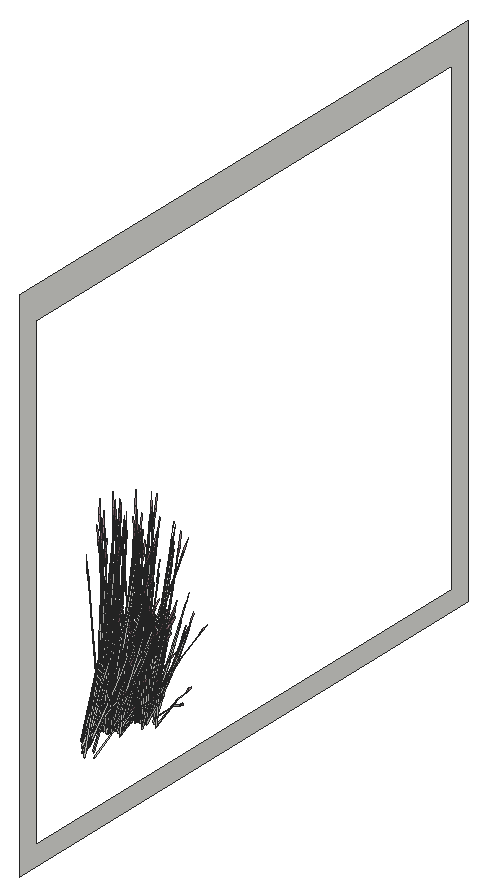
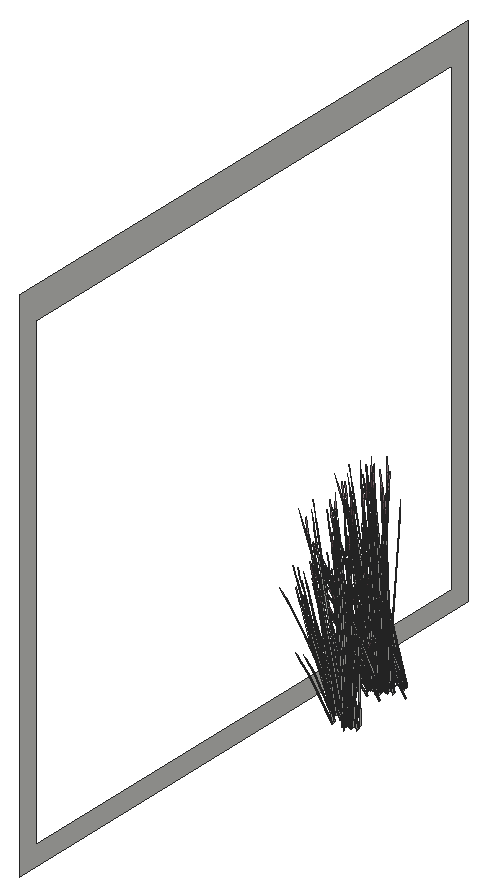
# SketchUp Ruby script. Lengths in inches.
U = 1.inch
M = Sketchup.active_model
def pt(a) = Geom::Point3d.new(a.map { |v| v * U })
def face(e, loops, mat)
  f = e.add_face(loops[0].map { |a| pt(a) })
  loops[1..].each { |l| e.add_face(l.map { |a| pt(a) }).erase! }
  f.material = f.back_material = mat if mat
  f
end
# faces: each face lists its corners as indices into pts; further lists are holes
def faces(e, pts, list, mat = nil) = list.each { |f| face(e, (f[0].is_a?(Array) ? f : [f]).map { |l| l.map { |i| pts[i] } }, mat) }
# xy, xz, yz: faces in a plane at the given z, y or x. An outline is a flat list of corners, or four numbers for a rectangle; further outlines are holes
def ring(l) = l.size == 4 ? [[l[0], l[1]], [l[2], l[1]], [l[2], l[3]], [l[0], l[3]]] : l.each_slice(2).to_a
def flat(e, list, mat, &to3) = list.each { |f| face(e, (f[0].is_a?(Array) ? f : [f]).map { |l| ring(l).map { |u, v| to3.(u, v) } }, mat) }
def xy(e, z, list, mat = nil) = flat(e, list, mat) { |x, y| [x, y, z] }
def xz(e, y, list, mat = nil) = flat(e, list, mat) { |x, z| [x, y, z] }
def yz(e, x, list, mat = nil) = flat(e, list, mat) { |y, z| [x, y, z] }
def lines(e, pts, list) = list.each { |a, b| e.add_line(pt(pts[a]), pt(pts[b])) }
# prism: a flat outline (further loops are holes) pulled along v
def prism(e, loops, v, mat = nil)
  f = face(e, loops, mat); d = Geom::Vector3d.new(v.map { |x| x * U })
  f.pushpull(f.normal.samedirection?(d) ? d.length : -d.length)
end
def box(e, o, s, mat = nil) = prism(e, [[o, [o[0] + s[0], o[1], o[2]], [o[0] + s[0], o[1] + s[1], o[2]], [o[0], o[1] + s[1], o[2]]]], [0, 0, s[2]], mat)
def at(x, y, z, deg = 0) = Geom::Transformation.translation(pt([x, y, z])) * Geom::Transformation.rotation(ORIGIN, Z_AXIS, deg.degrees)
def axes(o, x, y, z) = Geom::Transformation.new([*x, 0, *y, 0, *z, 0, *pt(o).to_a, 1])
def part(name) = M.definitions.add(name)
# library, detail: a bought-in or finely detailed component or shape, given as its bounding box
def library(name, o, s) = part(name).tap { |d| box(d.entities, o, s) }
def detail(e, o, s) = box(e.add_group.entities, o, s)
def put(e, d, t, mat = nil) = e.add_instance(d, t).tap { |i| i.material = mat if mat }
def group(e, t, mat = nil) = e.add_group.tap { |g| g.transformation = t; g.material = mat if mat }.entities
root = M.entities
M.materials.add("LightPink_Translucent").color = [144, 107, 117]
M.materials["LightPink_Translucent"].alpha = 0.75
c1 = part("blade")
p = [[2.15,0.21,22],[0,0.17,0],[0.09,0.45,0],[2.18,0.31,22],[2.29,0.31,22],[0.38,0.45,0],
  [2.48,0.24,33],[2.49,0.24,33],[2.48,0.22,33]]
faces(c1.entities,p,[[0,1,2,3],[4,5,2,3],[6,3,4,7],[8,0,3,6]])
c2 = part("seeds")
p = [[0.3,-0.1,1.38],[-0.01,-0.03,1.59],[-0.01,-0.03,0.03],[0.14,-0.07,-0.07],[0.29,-0.03,3],[0.15,0.01,3.11]]
faces(c2.entities,p,[[0,1,2,3],[1,0,4,5]],"LightPink_Translucent")
c3 = part("blade with seeds")
put(c3.entities,c1,at(0,0,0))
put(c3.entities,c2,axes([2.4,0.25,30.99],[1.5799,-0.05474,1.17369],[-0.12525,1.92788,0.29478],[-0.07173,-0.02425,1.56792]))
yz(root,366,[[[45,0,219,162],[51,6,213,151.99]]])
put(root,c3,axes([347.85,102.97,10.68],[-0.22982,-0.59576,-0.51099],[0.87033,-0.10422,-0.3958],[0.24941,-0.16002,0.97773]))
put(root,c3,axes([344.8,97.15,7],[0.00265,-0.07899,1.77383],[0.76665,-0.34851,-0.16761],[0.2663,0.12439,0.31391]))
put(root,c3,axes([347.41,96.85,3.79],[0.06518,-0.0942,1.76342],[0.82057,-0.27742,-0.26939],[0.24877,0.14358,0.30037]))
put(root,c3,axes([346.33,94.71,4.39],[0.32803,0.59738,-0.69212],[-0.94492,0.21515,-0.18165],[0.03626,0.20229,1.52773]))
put(root,c3,axes([346.13,96.41,6.97],[0.88277,-0.1551,-0.51099],[0.15442,0.58737,-0.3958],[0.23711,0.16832,0.97773]))
put(root,c3,axes([343.68,96.5,7.34],[0.2697,-0.50175,0.35414],[0.78684,0.14635,-0.4572],[0.07215,0.20201,0.87481]))
put(root,c3,axes([347.35,97,4.96],[-0.57368,-0.02046,1.0506],[0.37886,-0.43461,0.58006],[0.22663,0.15441,0.8241]))
put(root,c3,axes([345.7,96.89,7.02],[-0.4066,0.41448,0.0643],[-0.57901,-0.24131,0.50621],[0.18719,0.13288,0.77189]))
put(root,c3,axes([343.58,101.61,8.02],[0.83726,-0.32623,-0.49651],[0.50045,0.58498,0],[0.19069,-0.0743,1.57504]))
put(root,c3,axes([344.74,98.29,7.9375],[0.61821,-0.37431,-0.06488],[0.56645,0.40995,-0.29416],[0.03988,0.11616,0.97024]))
put(root,c3,axes([348.55,102.74,8.59],[-0.31959,-0.01933,1.43002],[-0.32741,-0.51843,-0.30754],[0.39262,-0.14666,0.61141]))
put(root,c3,axes([345.87,96.77,7.03],[-0.88979,0.14973,0.48003],[-0.15442,-0.58737,0.3958],[0.20926,0.17311,0.9933]))
put(root,c3,axes([344.57,102.95,8.06],[0.60257,-0.49041,-0.62353],[0.74854,0.44469,-0.16365],[0.24146,-0.12234,1.37633]))
put(root,c3,axes([348.92,101.79,8.77],[-0.29798,0.33213,1.1486],[-0.25612,-0.44624,0.84392],[0.24611,-0.11182,0.25299]))
put(root,c3,axes([345.48,95.95,4.88],[0.01579,-0.21629,1.43002],[0.75442,-0.24159,-0.30754],[0.23289,0.25887,0.61141]))
put(root,c3,axes([348.49,103.04,10.53],[0.77872,-0.09325,-0.35414],[0.20563,0.53305,0.4572],[0.22316,-0.14318,0.87481]))
put(root,c3,axes([343.42,96.71,7.33],[0.87543,-0.30377,-0.1216],[0.4302,0.53915,-0.67495],[0.1155,0.2272,1.02557]))
put(root,c3,axes([343.53,103.8125,8.21],[0.43405,-0.58792,-0.44739],[0.90188,0.28295,0.21531],[0,-0.13553,1.43643]))
put(root,c3,axes([343.92,103.52,8.67],[-0.10425,-0.7445,-0.29095],[1.08575,-0.04502,-0.50002],[0.19119,-0.09917,1.59708]))
put(root,c3,axes([343.58,96.83,3.79],[0.14478,-0.0355,1.76342],[0.8709,0.19542,-0.26939],[0.02547,0.22025,0.30037]))
put(root,c3,axes([343.78,101.87,8.03],[0.83462,0.16144,-0.30978],[-0.21015,0.56852,0.30978],[0.16826,-0.06556,1.38974]))
put(root,c3,axes([344.17,96.68,6.97],[0.87941,0.16356,-0.51099],[-0.30143,0.56078,-0.3958],[0.08064,0.22578,0.97773]))
put(root,c3,axes([344.67,95.52,6.17],[-0.2045,-0.20949,1.71376],[0.94495,-0.17636,0.13857],[0.21357,0.32887,0.73262]))
put(root,c3,axes([343.77,97.03,6.82],[-0.2697,0.50175,-0.35414],[-0.78684,-0.14635,0.4572],[0.07215,0.20201,0.87481]))
put(root,c3,axes([344.0625,104.1,8.43],[1.00799,0.31623,0.24065],[-0.48511,0.65709,0.50002],[0,-0.15147,1.60543]))
put(root,c3,axes([343.85,96.58,7.27],[0.42698,0.53052,-0.71045],[-0.87893,0.29566,0.08574],[0.09984,0.25633,1.00501]))
put(root,c3,axes([343.21,97.92,7.01],[0.1134,0.10507,1.74944],[0.91515,0.04128,-0.27667],[0.09203,0.23172,0.14031]))
put(root,c3,axes([343.74,103.66,8.72],[-0.97146,0.04028,0.44739],[-0.08785,-0.66859,-0.21531],[0.17391,-0.06776,1.43643]))
put(root,c3,axes([348.26,104.3,10.68],[0.24236,-0.59349,-0.51099],[0.83094,0.20343,-0.3958],[0.33455,-0.05442,0.97773]))
put(root,c3,axes([346.94,101.88,8.375],[0.55932,-0.6538,0],[0.93577,0.36461,-0.51607],[0.21313,0.08304,1.63711]))
put(root,c3,axes([349.14,104.46,7.98],[-0.57619,0.0783,1.41583],[-0.09171,-0.62326,0.08104],[0.40356,-0.09434,0.80566]))
put(root,c3,axes([350.19,103.91,8.26],[-0.55463,-0.41721,-0.06488],[0.60744,-0.38228,-0.29416],[0.17212,-0.02691,0.97024]))
put(root,c3,axes([345.1,103.97,8.21],[0,-0.75495,0],[1.11865,0,0],[0,0,1.79456]))
put(root,c3,axes([346.46,102.22,8.48],[-0.83726,-0.32623,0.49651],[0.50045,-0.58498,0],[0.19069,0.0743,1.57504]))
put(root,c3,axes([348.1,104.51,10.98],[0.78611,-0.28816,-0.71045],[0.4381,0.59317,0.08574],[0.37982,-0.06738,1.00501]))
put(root,c3,axes([344.57,103.49,8.36],[-0.74176,0.59212,0.45755],[-0.88124,-0.52269,0.17955],[0.17882,-0.05909,1.58856]))
put(root,c3,axes([343.29,102.52,8.47],[-0.25843,0.64844,0.17642],[-0.9457,-0.1835,0.35086],[0.16336,-0.00316,1.60407]))
put(root,c3,axes([342.89,103.04,7.59],[-0.88056,0.26122,1.28929],[-0.28027,-0.74951,0.50096],[0.54072,0.01247,1.46642]))
put(root,c3,axes([345.26,103.24,8.62],[0.17258,-0.58229,0.1448],[0.84319,0.10108,-0.41347],[0.15345,0.05979,1.26744]))
put(root,c3,axes([349.77,104.06,7.49],[-0.04675,-0.09906,1.76342],[0.32428,-0.57943,-0.26939],[0.32711,-0.00833,0.30037]))
put(root,c3,axes([344.9,103.39,8.72],[-0.53742,-0.54764,0.44739],[0.81403,-0.38564,-0.21531],[0.17391,0.06776,1.43643]))
put(root,c3,axes([345.17,103.43,8.67],[0.90324,-0.43318,-0.29095],[0.60064,0.61207,-0.50002],[0.22285,0.06216,1.59708]))
put(root,c3,axes([348.76,104.57,10.53],[0.74348,0.18202,-0.35414],[-0.21685,0.53102,0.4572],[0.29933,-0.04869,0.87481]))
put(root,c3,axes([347.45,102.27,8.02],[0.83726,0.32623,-0.49651],[-0.50045,0.58498,0],[0.19069,0.0743,1.57504]))
put(root,c3,axes([345.86,104.14,8.21],[1.00089,0,0],[0,0.67548,0],[0,0,1.78407]))
put(root,c3,axes([346.15,102.55,8.47],[-0.96132,0.17317,0.17642],[-0.23737,-0.64447,0.35086],[0.08574,0.0939,1.60407]))
put(root,c3,axes([346.74,103.91,9.875],[-0.37107,0.01478,1.71376],[0.24616,-0.64047,0.13857],[0.5288,0.03961,0.73262]))
put(root,c3,axes([347.22,102.52,8.03],[0.21015,0.56852,-0.30978],[-0.83462,0.16144,0.30978],[0.16826,0.06556,1.38974]))
put(root,c3,axes([345.54,103.79,8.38],[-1.13071,-0.13747,0.49198],[0.23011,-0.77639,0.19306],[0.16524,0.07497,1.70813]))
put(root,c3,axes([344.64,105.71,8.2],[-0.29189,-0.56252,0],[0.83351,-0.19699,0],[0,0,1.54371]))
put(root,c3,axes([345.73,105.63,8.18],[0.93921,-0.22138,-0.19198],[0.33003,0.6377,0.00008],[0.10367,-0.02447,1.73897]))
put(root,c3,axes([345.84,104.43,8.21],[0.62448,0.42144,0],[-0.62448,0.42144,0],[0,0,1.69266]))
put(root,c3,axes([347.53,104.24,8.47],[-0.70288,-0.47526,0.17642],[0.70832,-0.46097,0.35086],[-0.07763,0.09706,1.60407]))
put(root,c3,axes([346.23,103.52,8.06],[0.9306,0.10697,-0.62353],[-0.19638,0.65984,-0.16365],[0.27771,0.07995,1.37633]))
put(root,c3,axes([350.34,104.68,8.77],[-0.55274,0.10771,1.1486],[0.26018,-0.44517,0.84392],[0.29323,0.03046,0.25299]))
put(root,c3,axes([345.83,103.93,8.72],[0.43405,-0.58792,0.44739],[0.90188,0.28295,-0.21531],[0,0.13553,1.43643]))
put(root,c3,axes([345.67,104.27,8.29],[0,0.75458,-0.05637],[-1.11865,0,0],[0,0.02371,1.79368]))
put(root,c3,axes([345.75,103.73,8.21],[0.53742,0.54764,-0.44739],[-0.81403,0.38564,0.21531],[0.17391,0.06776,1.43643]))
put(root,c3,axes([349.38,106.05,9.93],[-0.17122,-0.54847,-0.03492],[0.80929,-0.12609,-0.15832],[0.169,0.03477,0.52218]))
put(root,c3,axes([348.11,104.26,8.48],[0,-0.65246,0.49651],[1.00089,0,0],[0,0.1486,1.57504]))
put(root,c3,axes([346.21,104.07,8.62],[0.83351,-0.19028,0.1448],[0.29189,0.54335,-0.41347],[0,0.11958,1.26744]))
put(root,c3,axes([349.31,105.39,8.59],[-0.21545,-0.16047,1.43002],[0.28033,-0.53085,-0.30754],[0.43591,0.07191,0.61141]))
put(root,c3,axes([345.45,105.97,8.2],[0.90188,0.29293,0],[-0.43405,0.60866,0],[0,0,1.74954]))
put(root,c3,axes([347.33,105.71,10.98],[0.89428,0.01571,-0.71045],[-0.06006,0.66153,0.08574],[0.37886,0.06981,1.00501]))
put(root,c3,axes([345.13,105.73,8.29],[0.38895,0.74956,-0.06012],[-1.11135,0.26265,0],[0.01358,0.02618,1.72173]))
put(root,c3,axes([348.79,104.37,8.375],[1.11865,0,0],[0,0.72922,-0.51607],[0,0.16609,1.63711]))
put(root,c3,axes([348.34,104.75,8.2],[-1.1181,-0.00522,-0.04976],[0,-0.72922,0.49943],[-0.03514,0.166,1.58352]))
put(root,c3,axes([345.92,104.11,8.67],[1.00749,0.31132,-0.29095],[-0.48511,0.65709,-0.50002],[0.03166,0.16133,1.59708]))
put(root,c3,axes([347.87,105.99,10.53],[0.50902,0.40851,-0.35414],[-0.58122,0.38671,0.4572],[0.29531,0.05884,0.87481]))
put(root,c3,axes([348.11,104.85,8.03],[-0.62448,0.40708,-0.30978],[-0.62448,-0.40708,0.30978],[0,0.13112,1.38974]))
put(root,c3,axes([345.81,104.6,8.21],[-0.43405,0.58792,-0.44739],[-0.90188,-0.28295,0.21531],[0,0.13553,1.43643]))
put(root,c3,axes([348.54,104.87,8.02],[0,0.65246,-0.49651],[-1.00089,0,0],[0,0.1486,1.57504]))
put(root,c3,axes([346.04,104.9375,9.875],[-0.3323,-0.11241,1.71376],[0.68769,-0.4716,0.13857],[0.42861,0.21275,0.73262]))
put(root,c3,axes([347.27,106.22,8.77],[-0.5037,-0.18761,1.1486],[0.6504,-0.19062,0.84392],[0.17543,0.16147,0.25299]))
put(root,c3,axes([347.41,106.92,7.49],[0.06518,-0.0942,1.76342],[0.82057,-0.27742,-0.26939],[0.24877,0.14358,0.30037]))
put(root,c3,axes([346.33,104.78,8.09],[0.32803,0.59738,-0.69212],[-0.94492,0.21515,-0.18165],[0.03626,0.20229,1.52773]))
put(root,c3,axes([346.13,106.48,10.68],[0.88277,-0.1551,-0.51099],[0.15442,0.58737,-0.3958],[0.23711,0.16832,0.97773]))
put(root,c3,axes([347.35,107.07,8.67],[-0.57368,-0.02046,1.0506],[0.37886,-0.43461,0.58006],[0.22663,0.15441,0.8241]))
put(root,c3,axes([346.1,115.19,4.88],[-0.25429,0.13207,1.43002],[-0.76157,-0.23115,-0.30754],[0.14117,-0.28747,0.61141]))
put(root,c3,axes([345.48,106.02,8.59],[0.01579,-0.21629,1.43002],[0.75442,-0.24159,-0.30754],[0.23289,0.25887,0.61141]))
put(root,c3,axes([346.72,116.17,7.27],[0.02328,-0.60353,-0.71045],[0.98022,0.04053,0.08574],[0.10344,-0.25568,1.00501]))
put(root,c3,axes([348.09,115.23,7.01],[-0.00864,-0.12985,1.74944],[-0.72937,-0.3753,-0.27667],[0.11277,-0.2275,0.14031]))
put(root,c3,axes([345.62,115.87,6.17],[-0.16657,0.22426,1.71376],[-0.69879,-0.4641,0.13857],[0.31524,-0.28926,0.73262]))
put(root,c3,axes([347.89,114.76,7],[-0.09085,0.04984,1.77383],[-0.89014,-0.16814,-0.16761],[-0.03222,-0.21748,0.31391]))
put(root,c3,axes([343.58,106.89,7.49],[0.14478,-0.0355,1.76342],[0.8709,0.19542,-0.26939],[0.02547,0.22025,0.30037]))
put(root,c3,axes([345.16,114.14,5.06],[0.11476,0.38047,1.1486],[-0.63664,-0.21072,0.84392],[0.06851,-0.19481,0.25299]))
put(root,c3,axes([344.17,106.75,10.68],[0.87941,0.16356,-0.51099],[-0.30143,0.56078,-0.3958],[0.08064,0.22578,0.97773]))
put(root,c3,axes([344.67,105.59,9.875],[-0.2045,-0.20949,1.71376],[0.94495,-0.17636,0.13857],[0.21357,0.32887,0.73262]))
put(root,c3,axes([346.52,115.97,6.97],[-0.64041,-0.4384,-0.51099],[0.67652,-0.38394,-0.3958],[0.09744,-0.22274,0.97773]))
put(root,c3,axes([343.77,107.09,10.53],[-0.2697,0.50175,-0.35414],[-0.78684,-0.14635,0.4572],[0.07215,0.20201,0.87481]))
put(root,c3,axes([345.12,115.32,7.03],[0.88151,0.17057,0.48003],[-0.30143,0.56078,0.3958],[-0.05297,-0.22053,0.9933]))
put(root,c3,axes([347.19,116.2,7.33],[-0.98321,-0.03233,-0.1216],[0.02687,-0.61208,-0.67495],[0.0683,-0.23574,1.02557]))
put(root,c3,axes([347.12,115.81,6.82],[0.60531,-0.34352,-0.35414],[0.573,0.39225,0.4572],[0.08718,-0.19929,0.87481]))
put(root,c3,axes([345.35,115.28,7.02],[0.6592,-0.22175,0.0643],[0.32265,0.40436,0.50621],[-0.06366,-0.17825,0.77189]))
put(root,c3,axes([343.85,106.64,10.98],[0.42698,0.53052,-0.71045],[-0.87893,0.29566,0.08574],[0.09984,0.25633,1.00501]))
put(root,c3,axes([347.88,115.6,3.79],[-0.1339,-0.0514,1.76342],[-0.34394,-0.57425,-0.26939],[0.23202,-0.15583,0.30037]))
put(root,c3,axes([347.12,115.94,7.03],[0.63704,0.44518,0.48003],[-0.67652,0.38394,0.3958],[0.11751,-0.20886,0.9933]))
put(root,c3,axes([347.36,115.99,7.02],[0.73517,0.0304,0.0643],[-0.02016,0.45906,0.50621],[0.07693,-0.17585,0.77189]))
put(root,c3,axes([346.81,116.3,7.34],[-0.60531,0.34352,0.35414],[-0.573,-0.39225,-0.4572],[0.08718,-0.19929,0.87481]))
put(root,c3,axes([347.875,117.22,7.27],[0.4673,-0.51481,-0.71045],[0.81887,0.36587,0.08574],[0.27902,-0.18652,1.00501]))
put(root,c3,axes([342.82,115.72,4.67],[-0.55932,-0.6538,0],[0.93577,-0.36461,-0.51607],[0.21313,-0.08304,1.63711]))
put(root,c3,axes([347.85,116.98,6.97],[-0.22982,-0.59576,-0.51099],[0.87033,-0.10422,-0.3958],[0.24941,-0.16002,0.97773]))
put(root,c3,axes([348.26,117.41,7.33],[-0.82753,-0.35977,-0.1216],[0.47675,-0.52101,-0.67495],[0.2338,-0.18111,1.02557]))
put(root,c3,axes([343.58,115.62,4.3125],[0.83726,-0.32623,-0.49651],[0.50045,0.58498,0],[0.19069,-0.0743,1.57504]))
put(root,c3,axes([348.55,116.75,4.88],[-0.31959,-0.01933,1.43002],[-0.32741,-0.51843,-0.30754],[0.39262,-0.14666,0.61141]))
put(root,c3,axes([350.3,117.25,7],[-0.11685,-0.00496,1.77383],[-0.48522,-0.53096,-0.16761],[0.19486,-0.17458,0.31391]))
put(root,c3,axes([344.57,116.96,4.35],[0.60257,-0.49041,-0.62353],[0.74854,0.44469,-0.16365],[0.24146,-0.12234,1.37633]))
put(root,c3,axes([348.92,115.8,5.06],[-0.29798,0.33213,1.1486],[-0.25612,-0.44624,0.84392],[0.24611,-0.11182,0.25299]))
put(root,c3,axes([348.49,117.04,6.82],[0.77872,-0.09325,-0.35414],[0.20563,0.53305,0.4572],[0.22316,-0.14318,0.87481]))
put(root,c3,axes([343.53,117.82,4.5],[0.43405,-0.58792,-0.44739],[0.90188,0.28295,0.21531],[0,-0.13553,1.43643]))
put(root,c3,axes([343.92,117.53,4.96],[-0.10425,-0.7445,-0.29095],[1.08575,-0.04502,-0.50002],[0.19119,-0.09917,1.59708]))
put(root,c3,axes([347.86,117.36,7.34],[-0.77872,0.09325,0.35414],[-0.20563,-0.53305,-0.4572],[0.22316,-0.14318,0.87481]))
put(root,c3,axes([343.78,115.88,4.32],[0.83462,0.16144,-0.30978],[-0.21015,0.56852,0.30978],[0.16826,-0.06556,1.38974]))
put(root,c3,axes([348.5625,117.27,7.02],[0.61415,0.2744,0.0643],[-0.35756,0.39076,0.50621],[0.1969,-0.12633,0.77189]))
put(root,c3,axes([348.39,117.16,7.03],[0.22187,0.60049,0.48003],[-0.87033,0.10422,0.3958],[0.25651,-0.14123,0.9933]))
put(root,c3,axes([350.74,117.89,7.01],[0.12414,-0.09938,1.74944],[-0.15889,-0.60963,-0.27667],[0.31148,-0.11559,0.14031]))
put(root,c3,axes([344.0625,118.11,4.73],[1.00799,0.31623,0.24065],[-0.48511,0.65709,0.50002],[0,-0.15147,1.60543]))
put(root,c3,axes([343.74,117.67,5.01],[-0.97146,0.04028,0.44739],[-0.08785,-0.66859,-0.21531],[0.17391,-0.06776,1.43643]))
put(root,c3,axes([348.29,118.8125,7.33],[-0.45012,-0.59081,-0.1216],[0.79888,-0.29033,-0.67495],[0.33665,-0.07795,1.02557]))
put(root,c3,axes([348.26,118.3,6.97],[0.24236,-0.59349,-0.51099],[0.83094,0.20343,-0.3958],[0.33455,-0.05442,0.97773]))
put(root,c3,axes([346.94,115.89,4.67],[0.55932,-0.6538,0],[0.93577,0.36461,-0.51607],[0.21313,0.08304,1.63711]))
put(root,c3,axes([349.14,118.47,4.28],[-0.57619,0.0783,1.41583],[-0.09171,-0.62326,0.08104],[0.40356,-0.09434,0.80566]))
put(root,c3,axes([350.19,117.92,4.55],[-0.55463,-0.41721,-0.06488],[0.60744,-0.38228,-0.29416],[0.17212,-0.02691,0.97024]))
put(root,c3,axes([345.1,117.97,4.5],[0,-0.75495,0],[1.11865,0,0],[0,0,1.79456]))
put(root,c3,axes([346.46,116.23,4.77],[-0.83726,-0.32623,0.49651],[0.50045,-0.58498,0],[0.19069,0.0743,1.57504]))
put(root,c3,axes([348.1,118.52,7.27],[0.78611,-0.28816,-0.71045],[0.4381,0.59317,0.08574],[0.37982,-0.06738,1.00501]))
put(root,c3,axes([344.57,117.5,4.65],[-0.74176,0.59212,0.45755],[-0.88124,-0.52269,0.17955],[0.17882,-0.05909,1.58856]))
put(root,c3,axes([343.29,116.52,4.77],[-0.25843,0.64844,0.17642],[-0.9457,-0.1835,0.35086],[0.16336,-0.00316,1.60407]))
put(root,c3,axes([347.98,118.63,7.34],[-0.74348,-0.18202,0.35414],[0.21685,-0.53102,-0.4572],[0.29933,-0.04869,0.87481]))
put(root,c3,axes([342.89,117.05,3.89],[-0.88056,0.26122,1.28929],[-0.28027,-0.74951,0.50096],[0.54072,0.01247,1.46642]))
put(root,c3,axes([345.26,117.24,4.91],[0.17258,-0.58229,0.1448],[0.84319,0.10108,-0.41347],[0.15345,0.05979,1.26744]))
put(root,c3,axes([349.77,118.06,3.79],[-0.04675,-0.09906,1.76342],[0.32428,-0.57943,-0.26939],[0.32711,-0.00833,0.30037]))
put(root,c3,axes([344.9,117.4,5.01],[-0.53742,-0.54764,0.44739],[0.81403,-0.38564,-0.21531],[0.17391,0.06776,1.43643]))
put(root,c3,axes([345.17,117.43,4.96],[0.90324,-0.43318,-0.29095],[0.60064,0.61207,-0.50002],[0.22285,0.06216,1.59708]))
put(root,c3,axes([348.76,118.58,6.82],[0.74348,0.18202,-0.35414],[-0.21685,0.53102,0.4572],[0.29933,-0.04869,0.87481]))
put(root,c3,axes([347.45,116.28,4.3125],[0.83726,0.32623,-0.49651],[-0.50045,0.58498,0],[0.19069,0.0743,1.57504]))
put(root,c3,axes([345.86,118.14,4.5],[1.00089,0,0],[0,0.67548,0],[0,0,1.78407]))
put(root,c3,axes([346.15,116.56,4.77],[-0.96132,0.17317,0.17642],[-0.23737,-0.64447,0.35086],[0.08574,0.0939,1.60407]))
put(root,c3,axes([346.74,117.92,6.17],[-0.37107,0.01478,1.71376],[0.24616,-0.64047,0.13857],[0.5288,0.03961,0.73262]))
put(root,c3,axes([347.22,116.53,4.32],[0.21015,0.56852,-0.30978],[-0.83462,0.16144,0.30978],[0.16826,0.06556,1.38974]))
put(root,c3,axes([348.66,118.8,7.02],[0.32857,0.44488,0.0643],[-0.59916,0.21775,0.50621],[0.26412,-0.04296,0.77189]))
put(root,c3,axes([345.54,117.8,4.67],[-1.13071,-0.13747,0.49198],[0.23011,-0.77639,0.19306],[0.16524,0.07497,1.70813]))
put(root,c3,axes([348.59,118.64,7.03],[-0.25275,0.59491,0.48003],[-0.83094,-0.20343,0.3958],[0.32677,-0.03575,0.9933]))
put(root,c3,axes([344.64,119.72,4.5],[-0.29189,-0.56252,0],[0.83351,-0.19699,0],[0,0,1.54371]))
